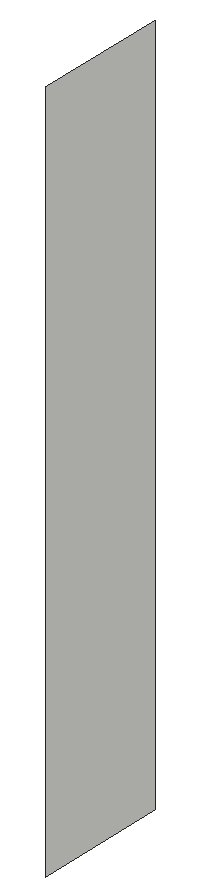
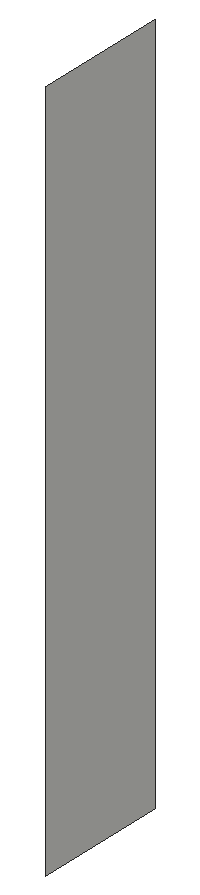
# SketchUp Ruby script. Lengths in inches.
U = 1.inch
M = Sketchup.active_model
def pt(a) = Geom::Point3d.new(a.map { |v| v * U })
def face(e, loops, mat)
  f = e.add_face(loops[0].map { |a| pt(a) })
  loops[1..].each { |l| e.add_face(l.map { |a| pt(a) }).erase! }
  f.material = f.back_material = mat if mat
  f
end
# faces: each face lists its corners as indices into pts; further lists are holes
def faces(e, pts, list, mat = nil) = list.each { |f| face(e, (f[0].is_a?(Array) ? f : [f]).map { |l| l.map { |i| pts[i] } }, mat) }
# xy, xz, yz: faces in a plane at the given z, y or x. An outline is a flat list of corners, or four numbers for a rectangle; further outlines are holes
def ring(l) = l.size == 4 ? [[l[0], l[1]], [l[2], l[1]], [l[2], l[3]], [l[0], l[3]]] : l.each_slice(2).to_a
def flat(e, list, mat, &to3) = list.each { |f| face(e, (f[0].is_a?(Array) ? f : [f]).map { |l| ring(l).map { |u, v| to3.(u, v) } }, mat) }
def xy(e, z, list, mat = nil) = flat(e, list, mat) { |x, y| [x, y, z] }
def xz(e, y, list, mat = nil) = flat(e, list, mat) { |x, z| [x, y, z] }
def yz(e, x, list, mat = nil) = flat(e, list, mat) { |y, z| [x, y, z] }
def lines(e, pts, list) = list.each { |a, b| e.add_line(pt(pts[a]), pt(pts[b])) }
# prism: a flat outline (further loops are holes) pulled along v
def prism(e, loops, v, mat = nil)
  f = face(e, loops, mat); d = Geom::Vector3d.new(v.map { |x| x * U })
  f.pushpull(f.normal.samedirection?(d) ? d.length : -d.length)
end
def box(e, o, s, mat = nil) = prism(e, [[o, [o[0] + s[0], o[1], o[2]], [o[0] + s[0], o[1] + s[1], o[2]], [o[0], o[1] + s[1], o[2]]]], [0, 0, s[2]], mat)
def at(x, y, z, deg = 0) = Geom::Transformation.translation(pt([x, y, z])) * Geom::Transformation.rotation(ORIGIN, Z_AXIS, deg.degrees)
def axes(o, x, y, z) = Geom::Transformation.new([*x, 0, *y, 0, *z, 0, *pt(o).to_a, 1])
def part(name) = M.definitions.add(name)
# library, detail: a bought-in or finely detailed component or shape, given as its bounding box
def library(name, o, s) = part(name).tap { |d| box(d.entities, o, s) }
def detail(e, o, s) = box(e.add_group.entities, o, s)
def put(e, d, t, mat = nil) = e.add_instance(d, t).tap { |i| i.material = mat if mat }
def group(e, t, mat = nil) = e.add_group.tap { |g| g.transformation = t; g.material = mat if mat }.entities
root = M.entities
yz(root,211.5,[[403.76,103.6875,424.53,211.6875]])
